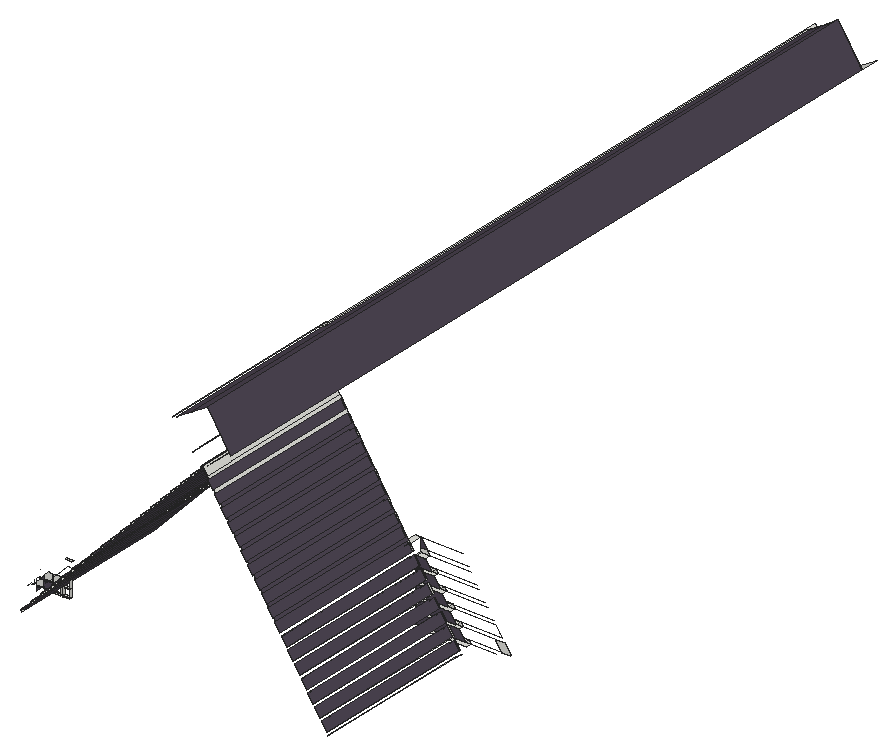
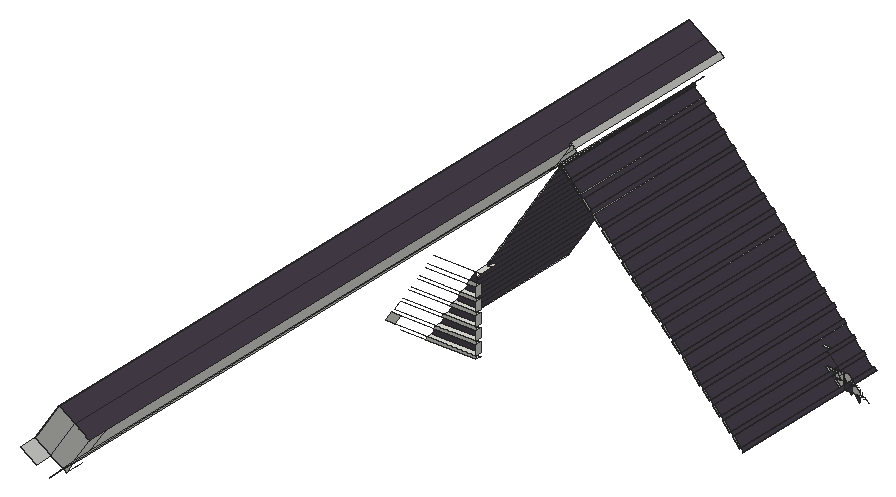
# SketchUp Ruby script. Lengths in inches.
U = 1.inch
M = Sketchup.active_model
def pt(a) = Geom::Point3d.new(a.map { |v| v * U })
def face(e, loops, mat)
  f = e.add_face(loops[0].map { |a| pt(a) })
  loops[1..].each { |l| e.add_face(l.map { |a| pt(a) }).erase! }
  f.material = f.back_material = mat if mat
  f
end
# faces: each face lists its corners as indices into pts; further lists are holes
def faces(e, pts, list, mat = nil) = list.each { |f| face(e, (f[0].is_a?(Array) ? f : [f]).map { |l| l.map { |i| pts[i] } }, mat) }
# xy, xz, yz: faces in a plane at the given z, y or x. An outline is a flat list of corners, or four numbers for a rectangle; further outlines are holes
def ring(l) = l.size == 4 ? [[l[0], l[1]], [l[2], l[1]], [l[2], l[3]], [l[0], l[3]]] : l.each_slice(2).to_a
def flat(e, list, mat, &to3) = list.each { |f| face(e, (f[0].is_a?(Array) ? f : [f]).map { |l| ring(l).map { |u, v| to3.(u, v) } }, mat) }
def xy(e, z, list, mat = nil) = flat(e, list, mat) { |x, y| [x, y, z] }
def xz(e, y, list, mat = nil) = flat(e, list, mat) { |x, z| [x, y, z] }
def yz(e, x, list, mat = nil) = flat(e, list, mat) { |y, z| [x, y, z] }
def lines(e, pts, list) = list.each { |a, b| e.add_line(pt(pts[a]), pt(pts[b])) }
# prism: a flat outline (further loops are holes) pulled along v
def prism(e, loops, v, mat = nil)
  f = face(e, loops, mat); d = Geom::Vector3d.new(v.map { |x| x * U })
  f.pushpull(f.normal.samedirection?(d) ? d.length : -d.length)
end
def box(e, o, s, mat = nil) = prism(e, [[o, [o[0] + s[0], o[1], o[2]], [o[0] + s[0], o[1] + s[1], o[2]], [o[0], o[1] + s[1], o[2]]]], [0, 0, s[2]], mat)
def at(x, y, z, deg = 0) = Geom::Transformation.translation(pt([x, y, z])) * Geom::Transformation.rotation(ORIGIN, Z_AXIS, deg.degrees)
def axes(o, x, y, z) = Geom::Transformation.new([*x, 0, *y, 0, *z, 0, *pt(o).to_a, 1])
def part(name) = M.definitions.add(name)
# library, detail: a bought-in or finely detailed component or shape, given as its bounding box
def library(name, o, s) = part(name).tap { |d| box(d.entities, o, s) }
def detail(e, o, s) = box(e.add_group.entities, o, s)
def put(e, d, t, mat = nil) = e.add_instance(d, t).tap { |i| i.material = mat if mat }
def group(e, t, mat = nil) = e.add_group.tap { |g| g.transformation = t; g.material = mat if mat }.entities
root = M.entities
M.materials.add("[Color M06]").color = [79, 71, 84]
xy(root,386.372,[[1096.787,2376.244,1113.36,2378.119]])
xy(root,386.399,[[1013.083,2332.135,1015.395,2332.76],[1015.995,2332.135,1018.307,2332.76]])
xy(root,386.837,[[1013.267,2332.135,1015.395,2332.76],[1015.995,2332.135,1018.307,2332.76]])
xy(root,387.495,[[1096.787,2376.244,1112.64,2378.119]])
xy(root,389.149,[[1015.995,2332.135,1018.307,2332.76]])
xy(root,389.587,[[1015.995,2332.135,1018.307,2332.76]])
xy(root,390.622,[[1096.787,2376.244,1110.635,2378.119]])
xy(root,391.745,[[1096.787,2376.244,1109.915,2378.119]])
xy(root,391.899,[[1018.012,2332.135,1018.307,2332.76]])
xy(root,394.872,[[1096.787,2376.244,1107.911,2378.119]])
xy(root,395.995,[[1096.787,2376.244,1107.191,2378.119]])
xy(root,397.749,[[1016.769,2332.135,1019.019,2332.76]])
xy(root,399.122,[[1096.787,2376.244,1105.186,2378.119]])
xy(root,400.245,[[1096.787,2376.244,1104.466,2378.119]])
xy(root,403.372,[[1096.787,2376.244,1102.461,2378.119]])
xy(root,404.495,[[1096.787,2376.244,1101.741,2378.119]])
xy(root,407.622,[[1096.787,2376.244,1099.736,2378.119]])
xy(root,412.223,[[1095.037,2371.682,1096.787,2373.557],[1095.037,2373.557,1096.787,2378.119]])
xz(root,2319.182,[[1073.488,447.754,1073.856,447.99,1072.287,450.4375,1071.978,450.109],[1071.978,450.109,1072.287,450.4375,1071.919,450.201]])
xz(root,2332.135,[[1007.259,385.926,1007.702,386.399,1007.259,386.399],[1010.171,386.283,1010.28,386.399,1010.171,386.399],[1006.497,386.837,1006.659,386.837,1006.659,387.008],[1007.259,386.837,1009.091,386.837,1009.571,387.346,1009.571,389.149,1008.674,389.149,1007.259,387.645],[1009.091,386.837,1009.571,386.837,1009.571,387.346],
  [1013.083,386.837,1013.267,386.837,1015.395,389.107,1015.395,389.149,1013.083,389.149],[1010.171,389.033,1010.28,389.149,1010.171,389.149],[1009.086,389.587,1009.571,389.587,1009.571,390.102],[1010.171,389.587,1011.68,389.587,1012.483,390.44,1012.483,391.899,1011.263,391.899,1010.171,390.739],[1011.68,389.587,1012.483,389.587,1012.483,390.44],
  [1013.083,389.587,1013.267,389.587,1015.395,391.857,1015.395,391.899,1013.857,391.899,1013.083,391.077],[1013.267,389.587,1015.395,389.587,1015.395,391.857],[1015.995,389.747,1018.012,391.899,1015.995,391.899],[1013.083,391.077,1013.857,391.899,1013.083,391.899]])
xz(root,2332.135,[[1007.259,384.89,1008.68,386.399,1007.702,386.399,1007.259,385.926],[1010.171,386.837,1012.483,386.837,1012.483,389.149,1011.268,389.149,1010.171,387.983,1009.571,387.346,1009.571,389.149,1008.674,389.149,1009.086,389.587,1009.571,389.587,1009.571,390.102,1010.171,390.739,1010.171,389.587,1011.68,389.587,1011.268,389.149,1010.171,389.149]],"[Color M06]")
xz(root,2371.682,[[1113.509,385.328,1113.453,385.417,1113.821,385.653,1113.878,385.565],[1111.317,388.748,1111.26,388.837,1111.628,389.073,1111.685,388.985],[1109.124,392.168,1109.068,392.257,1109.436,392.493,1109.493,392.405],[1106.932,395.588,1106.875,395.677,1107.243,395.913,1107.3,395.825],[1104.739,399.009,1104.682,399.097,1105.051,399.333,1105.107,399.245],
  [1102.547,402.429,1102.49,402.517,1102.858,402.753,1102.915,402.665],[1100.354,405.849,1100.297,405.937,1100.665,406.173,1100.722,406.085],[1098.161,409.269,1098.105,409.357,1098.473,409.593,1098.53,409.505],[1095.969,412.689,1095.912,412.777,1096.28,413.013,1096.337,412.925],[1093.776,416.109,1093.719,416.197,1094.088,416.433,1094.144,416.345],
  [1091.584,419.529,1091.527,419.617,1091.895,419.853,1091.952,419.765],[1089.391,422.949,1089.334,423.037,1089.702,423.273,1089.759,423.185],[1087.198,426.369,1087.142,426.457,1087.51,426.693,1087.567,426.605],[1085.006,429.789,1084.949,429.877,1085.317,430.113,1085.374,430.025],[1082.813,433.209,1082.756,433.297,1083.125,433.533,1083.181,433.445],
  [1080.621,436.629,1080.564,436.717,1080.932,436.953,1080.989,436.865],[1078.428,440.049,1078.371,440.137,1078.74,440.373,1078.796,440.285],[1076.235,443.469,1076.179,443.557,1076.547,443.793,1076.604,443.705],[1074.043,446.889,1073.986,446.977,1074.354,447.213,1074.411,447.125]])
xz(root,2373.557,[[1112.955,386.194,1111.317,388.748,1111.685,388.985,1113.323,386.43],[1013.667,387.25,1016.089,389.822,1015.633,390.251,1013.212,387.679],[1110.762,389.614,1109.124,392.168,1109.493,392.405,1111.13,389.85],[1016.966,390.754,1019.387,393.327,1018.932,393.755,1016.511,391.183],[1108.569,393.034,1106.932,395.588,1107.3,395.825,1108.938,393.27],
  [1020.265,394.259,1022.686,396.831,1022.231,397.259,1019.809,394.687],[1106.377,396.454,1104.739,399.009,1105.107,399.245,1106.745,396.69],[1023.563,397.763,1025.984,400.335,1025.529,400.763,1023.108,398.191],[1104.184,399.874,1102.547,402.429,1102.915,402.665,1104.553,400.11],[1026.862,401.267,1029.283,403.839,1028.828,404.268,1026.407,401.696],
  [1101.992,403.294,1100.354,405.849,1100.722,406.085,1102.36,403.53],[1030.16,404.771,1032.581,407.344,1032.126,407.772,1029.705,405.2],[1099.799,406.714,1098.161,409.269,1098.53,409.505,1100.167,406.95],[1033.459,408.276,1035.88,410.848,1035.425,411.276,1033.004,408.704],[1097.606,410.134,1096.419,411.987,1096.787,412.223,1097.975,410.37],
  [1036.757,411.78,1039.178,414.352,1038.723,414.78,1036.302,412.208],[1096.419,411.987,1096.267,412.223,1096.787,412.223],[1096.267,412.223,1096.787,412.223,1096.337,412.925,1095.969,412.689],[1095.414,413.554,1095.782,413.79,1094.594,415.643,1094.226,415.407],[1040.056,415.284,1042.477,417.856,1042.022,418.285,1039.601,415.713],
  [1094.226,415.407,1094.594,415.643,1094.144,416.345,1093.776,416.109],[1093.221,416.974,1093.59,417.21,1092.402,419.063,1092.033,418.827],[1043.354,418.788,1045.775,421.361,1045.32,421.789,1042.899,419.217],[1092.033,418.827,1092.402,419.063,1091.952,419.765,1091.584,419.529],[1091.029,420.394,1091.397,420.63,1090.209,422.483,1089.841,422.247],
  [1089.841,422.247,1090.209,422.483,1089.759,423.185,1089.391,422.949],[1046.653,422.293,1049.074,424.865,1048.619,425.293,1046.198,422.721],[1088.836,423.814,1089.204,424.05,1088.017,425.903,1087.648,425.667],[1087.648,425.667,1088.017,425.903,1087.567,426.605,1087.198,426.369],[1049.951,425.797,1052.373,428.369,1051.917,428.797,1049.496,426.225],
  [1086.643,427.234,1087.012,427.47,1085.824,429.323,1085.456,429.087],[1085.456,429.087,1085.824,429.323,1085.374,430.025,1085.006,429.789],[1053.25,429.301,1055.671,431.873,1055.216,432.302,1052.795,429.73],[1084.451,430.654,1084.819,430.89,1083.631,432.743,1083.263,432.507],[1083.263,432.507,1083.631,432.743,1083.181,433.445,1082.813,433.209],
  [1056.549,432.805,1058.97,435.378,1058.515,435.806,1056.093,433.234],[1082.258,434.074,1082.627,434.31,1081.439,436.163,1081.07,435.927],[1081.07,435.927,1081.439,436.163,1080.989,436.865,1080.621,436.629],[1059.847,436.31,1062.268,438.882,1061.813,439.31,1059.392,436.738],[1080.066,437.494,1080.434,437.73,1079.246,439.583,1078.878,439.347],
  [1078.878,439.347,1079.246,439.583,1078.796,440.285,1078.428,440.049],[1063.146,439.814,1065.567,442.386,1065.112,442.814,1062.69,440.242],[1077.873,440.914,1078.241,441.15,1077.054,443.003,1076.685,442.767],[1076.685,442.767,1077.054,443.003,1076.604,443.705,1076.235,443.469],[1066.444,443.318,1068.865,445.89,1068.41,446.319,1065.989,443.747],
  [1075.68,444.334,1076.049,444.57,1074.861,446.423,1074.493,446.187],[1074.493,446.187,1074.861,446.423,1074.411,447.125,1074.043,446.889],[1069.743,446.822,1072.164,449.395,1071.709,449.823,1069.288,447.251],[1073.488,447.754,1073.856,447.99,1072.668,449.843,1072.3,449.607],[1072.3,449.607,1072.668,449.843,1072.287,450.4375,1071.978,450.109],
  [1071.978,450.109,1071.919,450.201,1072.287,450.4375]])
xz(root,2376.244,[[1096.787,387.495,1112.64,387.495,1110.635,390.622,1096.787,390.622],[1096.787,391.745,1109.915,391.745,1107.911,394.872,1096.787,394.872],[1096.787,395.995,1107.191,395.995,1105.186,399.122,1096.787,399.122],[1096.787,400.245,1104.466,400.245,1102.461,403.372,1096.787,403.372],[1096.787,404.495,1101.741,404.495,1099.736,407.622,1096.787,407.622]],"[Color M06]")
xz(root,2378.119,[[1096.787,386.372,1113.36,386.372,1112.64,387.495,1096.787,387.495],[1123.539,387.495,1126.264,387.495,1124.259,390.622,1121.534,390.622],[1096.787,390.622,1110.635,390.622,1109.915,391.745,1096.787,391.745],[1096.787,394.872,1107.911,394.872,1107.191,395.995,1096.787,395.995],[1096.787,399.122,1105.186,399.122,1104.466,400.245,1096.787,400.245],
  [1096.787,403.372,1102.461,403.372,1101.741,404.495,1096.787,404.495],[1096.787,407.622,1099.736,407.622,1098.856,408.995,1096.787,408.995],[1096.787,412.122,1096.851,412.122,1096.787,412.223]])
xz(root,2378.119,[[1096.787,408.995,1098.856,408.995,1096.851,412.122,1096.787,412.122]],"[Color M06]")
xz(root,2380.477,[[1069.147,453.393,1061.61,460.488,1062.381,461.307,1066.649,457.29],[1069.147,453.393,1066.649,457.29,1069.918,454.213],[1069.918,454.213,1066.649,457.29,1067.977,458.7,1071.246,455.623],[1066.649,457.29,1062.381,461.307,1063.709,462.718,1067.977,458.7]])
xz(root,2571.585,[[1069.093,453.336,1069.147,453.393,1069.082,453.352]])
xz(root,2578.119,[[1071.34,449.83,1069.093,453.336,1069.147,453.393,1072.287,450.4375],[1072.287,450.4375,1069.147,453.393,1063.728,461.846,1068.662,465.009,1076.339,453.035],[1076.339,453.035,1068.662,465.009,1073.923,468.382,1081.6,456.408],[1069.093,453.336,1069.082,453.352,1069.147,453.393]])
yz(root,1015.395,[[2332.135,386.837,2332.76,389.107]])
yz(root,1015.995,[[2332.135,386.837,2332.76,389.149],[2332.135,389.587,2332.76,389.747]])
yz(root,1018.307,[[2332.135,386.837,2332.76,389.149],[2332.135,389.587,2332.76,391.899]])
yz(root,1096.787,[[2376.244,387.495,2378.119,390.622],[2376.244,391.745,2378.119,394.872],[2376.244,395.995,2378.119,399.122],[2376.244,400.245,2378.119,403.372],[2376.244,404.495,2378.119,407.622]])
p = [[1113.878,2371.682,385.565],[1113.878,2373.557,385.565],[1113.509,2373.557,385.328],[1113.509,2371.682,385.328],[1113.821,2319.182,385.653],[1113.821,2371.682,385.653],
  [1113.453,2371.682,385.417],[1113.453,2319.182,385.417],[1111.26,2319.182,388.837],[1111.26,2371.682,388.837],[1111.317,2371.682,388.748],[1111.317,2373.557,388.748],
  [1112.955,2373.557,386.194],[1112.955,2319.182,386.194],[1113.323,2373.557,386.43],[1113.323,2319.182,386.43],[1012.335,2373.557,386.746],[1012.335,2319.182,386.746],
  [1012.79,2319.182,386.318],[1012.79,2373.557,386.318],[1013.212,2373.557,387.679],[1013.212,2319.182,387.679],[1015.395,2332.135,389.107],[1013.267,2332.135,386.837],
  [1013.267,2332.76,386.837],[1015.395,2332.76,389.107],[1013.667,2373.557,387.25],[1013.667,2319.182,387.25],[1016.089,2373.557,389.822],[1016.089,2319.182,389.822],
  [1111.685,2371.682,388.985],[1111.685,2373.557,388.985],[1111.628,2319.182,389.073],[1111.628,2371.682,389.073],[1109.068,2319.182,392.257],[1109.068,2371.682,392.257],
  [1109.124,2371.682,392.168],[1109.124,2373.557,392.168],[1110.762,2373.557,389.614],[1110.762,2319.182,389.614],[1111.13,2373.557,389.85],[1111.13,2319.182,389.85],
  [1018.012,2332.135,391.899],[1015.995,2332.135,389.747],[1015.995,2332.76,389.747],[1018.012,2332.76,391.899],[1015.633,2373.557,390.251],[1015.633,2319.182,390.251],
  [1016.511,2373.557,391.183],[1016.511,2319.182,391.183],[1016.966,2373.557,390.754],[1016.966,2319.182,390.754],[1019.387,2373.557,393.327],[1019.387,2319.182,393.327],
  [1109.493,2371.682,392.405],[1109.493,2373.557,392.405],[1109.436,2319.182,392.493],[1109.436,2371.682,392.493],[1106.875,2319.182,395.677],[1106.875,2371.682,395.677],
  [1106.932,2371.682,395.588],[1106.932,2373.557,395.588],[1108.569,2373.557,393.034],[1108.569,2319.182,393.034],[1108.938,2373.557,393.27],[1108.938,2319.182,393.27],
  [1018.932,2373.557,393.755],[1018.932,2319.182,393.755],[1019.809,2373.557,394.687],[1019.809,2319.182,394.687],[1020.265,2373.557,394.259],[1020.265,2319.182,394.259],
  [1022.686,2373.557,396.831],[1022.686,2319.182,396.831],[1107.3,2371.682,395.825],[1107.3,2373.557,395.825],[1107.243,2319.182,395.913],[1107.243,2371.682,395.913],
  [1104.682,2319.182,399.097],[1104.682,2371.682,399.097],[1104.739,2371.682,399.009],[1104.739,2373.557,399.009],[1106.377,2373.557,396.454],[1106.377,2319.182,396.454],
  [1106.745,2373.557,396.69],[1106.745,2319.182,396.69],[1022.231,2373.557,397.259],[1022.231,2319.182,397.259],[1023.108,2373.557,398.191],[1023.108,2319.182,398.191],
  [1023.563,2373.557,397.763],[1023.563,2319.182,397.763],[1025.984,2373.557,400.335],[1025.984,2319.182,400.335],[1105.107,2371.682,399.245],[1105.107,2373.557,399.245],
  [1105.051,2319.182,399.333],[1105.051,2371.682,399.333],[1102.49,2319.182,402.517],[1102.49,2371.682,402.517],[1102.547,2371.682,402.429],[1102.547,2373.557,402.429],
  [1104.184,2373.557,399.874],[1104.184,2319.182,399.874],[1104.553,2373.557,400.11],[1104.553,2319.182,400.11],[1025.529,2373.557,400.763],[1025.529,2319.182,400.763],
  [1026.407,2373.557,401.696],[1026.407,2319.182,401.696],[1026.862,2373.557,401.267],[1026.862,2319.182,401.267],[1029.283,2373.557,403.839],[1029.283,2319.182,403.839],
  [1102.915,2371.682,402.665],[1102.915,2373.557,402.665],[1102.858,2319.182,402.753],[1102.858,2371.682,402.753],[1100.297,2319.182,405.937],[1100.297,2371.682,405.937],
  [1100.354,2371.682,405.849],[1100.354,2373.557,405.849],[1101.992,2373.557,403.294],[1101.992,2319.182,403.294],[1102.36,2373.557,403.53],[1102.36,2319.182,403.53],
  [1028.828,2373.557,404.268],[1028.828,2319.182,404.268],[1029.705,2373.557,405.2],[1029.705,2319.182,405.2],[1030.16,2373.557,404.771],[1030.16,2319.182,404.771],
  [1032.581,2373.557,407.344],[1032.581,2319.182,407.344],[1100.722,2371.682,406.085],[1100.722,2373.557,406.085],[1100.665,2319.182,406.173],[1100.665,2371.682,406.173],
  [1098.105,2319.182,409.357],[1098.105,2371.682,409.357],[1098.161,2371.682,409.269],[1098.161,2373.557,409.269],[1099.799,2373.557,406.714],[1099.799,2319.182,406.714],
  [1100.167,2373.557,406.95],[1100.167,2319.182,406.95],[1032.126,2373.557,407.772],[1032.126,2319.182,407.772],[1033.004,2373.557,408.704],[1033.004,2319.182,408.704],
  [1033.459,2373.557,408.276],[1033.459,2319.182,408.276],[1035.88,2373.557,410.848],[1035.88,2319.182,410.848],[1098.53,2371.682,409.505],[1098.53,2373.557,409.505],
  [1098.473,2319.182,409.593],[1098.473,2371.682,409.593],[1095.912,2319.182,412.777],[1095.912,2371.682,412.777],[1095.969,2371.682,412.689],[1095.969,2373.557,412.689],
  [1096.267,2373.557,412.223],[1096.419,2373.557,411.987],[1097.606,2373.557,410.134],[1097.606,2319.182,410.134],[1097.975,2373.557,410.37],[1097.975,2319.182,410.37],
  [1035.425,2373.557,411.276],[1035.425,2319.182,411.276],[1036.302,2373.557,412.208],[1036.302,2319.182,412.208],[1036.757,2373.557,411.78],[1036.757,2319.182,411.78],
  [1039.178,2373.557,414.352],[1039.178,2319.182,414.352],[1096.337,2371.682,412.925],[1096.337,2373.557,412.925],[1096.28,2319.182,413.013],[1096.28,2371.682,413.013],
  [1095.782,2319.182,413.79],[1095.782,2373.557,413.79],[1093.719,2319.182,416.197],[1093.719,2371.682,416.197],[1093.776,2371.682,416.109],[1093.776,2373.557,416.109],
  [1094.226,2373.557,415.407],[1095.414,2373.557,413.554],[1095.414,2319.182,413.554],[1038.723,2373.557,414.78],[1038.723,2319.182,414.78],[1039.601,2373.557,415.713],
  [1039.601,2319.182,415.713],[1040.056,2373.557,415.284],[1040.056,2319.182,415.284],[1042.477,2373.557,417.856],[1042.477,2319.182,417.856],[1094.144,2371.682,416.345],
  [1094.144,2373.557,416.345],[1094.088,2319.182,416.433],[1094.088,2371.682,416.433],[1093.59,2319.182,417.21],[1093.59,2373.557,417.21],[1091.527,2319.182,419.617],
  [1091.527,2371.682,419.617],[1091.584,2371.682,419.529],[1091.584,2373.557,419.529],[1092.033,2373.557,418.827],[1093.221,2373.557,416.974],[1093.221,2319.182,416.974],
  [1042.022,2373.557,418.285],[1042.022,2319.182,418.285],[1042.899,2373.557,419.217],[1042.899,2319.182,419.217],[1043.354,2373.557,418.788],[1043.354,2319.182,418.788],
  [1045.775,2373.557,421.361],[1045.775,2319.182,421.361],[1091.952,2371.682,419.765],[1091.952,2373.557,419.765],[1091.895,2319.182,419.853],[1091.895,2371.682,419.853],
  [1091.397,2319.182,420.63],[1091.397,2373.557,420.63],[1089.334,2319.182,423.037],[1089.334,2371.682,423.037],[1089.391,2371.682,422.949],[1089.391,2373.557,422.949],
  [1089.841,2373.557,422.247],[1091.029,2373.557,420.394],[1091.029,2319.182,420.394],[1045.32,2373.557,421.789],[1045.32,2319.182,421.789],[1046.198,2373.557,422.721],
  [1046.198,2319.182,422.721],[1046.653,2373.557,422.293],[1046.653,2319.182,422.293],[1049.074,2373.557,424.865],[1049.074,2319.182,424.865],[1089.759,2371.682,423.185],
  [1089.759,2373.557,423.185],[1089.702,2319.182,423.273],[1089.702,2371.682,423.273],[1089.204,2319.182,424.05],[1089.204,2373.557,424.05],[1087.142,2319.182,426.457],
  [1087.142,2371.682,426.457],[1087.198,2371.682,426.369],[1087.198,2373.557,426.369],[1087.648,2373.557,425.667],[1088.836,2373.557,423.814],[1088.836,2319.182,423.814],
  [1048.619,2373.557,425.293],[1048.619,2319.182,425.293],[1049.496,2373.557,426.225],[1049.496,2319.182,426.225],[1049.951,2373.557,425.797],[1049.951,2319.182,425.797],
  [1052.373,2373.557,428.369],[1052.373,2319.182,428.369],[1087.567,2371.682,426.605],[1087.567,2373.557,426.605],[1087.51,2319.182,426.693],[1087.51,2371.682,426.693],
  [1087.012,2319.182,427.47],[1087.012,2373.557,427.47],[1084.949,2319.182,429.877],[1084.949,2371.682,429.877],[1085.006,2371.682,429.789],[1085.006,2373.557,429.789],
  [1085.456,2373.557,429.087],[1086.643,2373.557,427.234],[1086.643,2319.182,427.234],[1051.917,2373.557,428.797],[1051.917,2319.182,428.797],[1052.795,2373.557,429.73],
  [1052.795,2319.182,429.73],[1053.25,2373.557,429.301],[1053.25,2319.182,429.301],[1055.671,2373.557,431.873],[1055.671,2319.182,431.873],[1085.374,2371.682,430.025],
  [1085.374,2373.557,430.025],[1085.317,2319.182,430.113],[1085.317,2371.682,430.113],[1084.819,2319.182,430.89],[1084.819,2373.557,430.89],[1082.756,2319.182,433.297],
  [1082.756,2371.682,433.297],[1082.813,2371.682,433.209],[1082.813,2373.557,433.209],[1083.263,2373.557,432.507],[1084.451,2373.557,430.654],[1084.451,2319.182,430.654],
  [1055.216,2373.557,432.302],[1055.216,2319.182,432.302],[1056.093,2373.557,433.234],[1056.093,2319.182,433.234],[1056.549,2373.557,432.805],[1056.549,2319.182,432.805],
  [1058.97,2373.557,435.378],[1058.97,2319.182,435.378],[1083.181,2371.682,433.445],[1083.181,2373.557,433.445],[1083.125,2319.182,433.533],[1083.125,2371.682,433.533],
  [1082.627,2319.182,434.31],[1082.627,2373.557,434.31],[1080.564,2319.182,436.717],[1080.564,2371.682,436.717],[1080.621,2371.682,436.629],[1080.621,2373.557,436.629],
  [1081.07,2373.557,435.927],[1082.258,2373.557,434.074],[1082.258,2319.182,434.074],[1058.515,2373.557,435.806],[1058.515,2319.182,435.806],[1059.392,2373.557,436.738],
  [1059.392,2319.182,436.738],[1059.847,2373.557,436.31],[1059.847,2319.182,436.31],[1062.268,2373.557,438.882],[1062.268,2319.182,438.882],[1080.989,2371.682,436.865],
  [1080.989,2373.557,436.865],[1080.932,2319.182,436.953],[1080.932,2371.682,436.953],[1080.434,2319.182,437.73],[1080.434,2373.557,437.73],[1078.371,2319.182,440.137],
  [1078.371,2371.682,440.137],[1078.428,2371.682,440.049],[1078.428,2373.557,440.049],[1078.878,2373.557,439.347],[1080.066,2373.557,437.494],[1080.066,2319.182,437.494],
  [1061.813,2373.557,439.31],[1061.813,2319.182,439.31],[1062.69,2373.557,440.242],[1062.69,2319.182,440.242],[1063.146,2373.557,439.814],[1063.146,2319.182,439.814],
  [1065.567,2373.557,442.386],[1065.567,2319.182,442.386],[1078.796,2371.682,440.285],[1078.796,2373.557,440.285],[1078.74,2319.182,440.373],[1078.74,2371.682,440.373],
  [1078.241,2319.182,441.15],[1078.241,2373.557,441.15],[1076.179,2319.182,443.557],[1076.179,2371.682,443.557],[1076.235,2371.682,443.469],[1076.235,2373.557,443.469],
  [1076.685,2373.557,442.767],[1077.873,2373.557,440.914],[1077.873,2319.182,440.914],[1065.112,2373.557,442.814],[1065.112,2319.182,442.814],[1065.989,2373.557,443.747],
  [1065.989,2319.182,443.747],[1066.444,2373.557,443.318],[1066.444,2319.182,443.318],[1068.865,2373.557,445.89],[1068.865,2319.182,445.89],[1076.604,2371.682,443.705],
  [1076.604,2373.557,443.705],[1076.547,2319.182,443.793],[1076.547,2371.682,443.793],[1076.049,2319.182,444.57],[1076.049,2373.557,444.57],[1073.986,2319.182,446.977],
  [1073.986,2371.682,446.977],[1074.043,2371.682,446.889],[1074.043,2373.557,446.889],[1074.493,2373.557,446.187],[1075.68,2373.557,444.334],[1075.68,2319.182,444.334],
  [1068.41,2373.557,446.319],[1068.41,2319.182,446.319],[1069.288,2373.557,447.251],[1069.288,2319.182,447.251],[1069.743,2373.557,446.822],[1069.743,2319.182,446.822],
  [1072.164,2373.557,449.395],[1072.164,2319.182,449.395],[1074.411,2371.682,447.125],[1074.411,2373.557,447.125],[1074.354,2319.182,447.213],[1074.354,2371.682,447.213],
  [1073.856,2319.182,447.99],[1073.856,2373.557,447.99],[1072.3,2373.557,449.607],[1073.488,2373.557,447.754],[1073.488,2319.182,447.754],[1071.978,2319.182,450.109],
  [1071.919,2319.182,450.201],[1071.919,2373.557,450.201],[1071.978,2373.557,450.109],[1072.668,2373.557,449.843],[1072.287,2373.557,450.4375],[1072.287,2319.182,450.4375],
  [1071.709,2373.557,449.823],[1071.709,2319.182,449.823],[1072.218,2373.557,450.545],[1072.162,2319.182,450.633],[1072.162,2371.682,450.633],[1072.218,2371.682,450.545],
  [1072.287,2380.477,450.4375],[1072.287,2571.585,450.4375],[1072.287,2578.119,450.4375],[1072.287,2583.74,450.4375],[1069.147,2583.74,453.393],[1069.147,2578.119,453.393],
  [1069.147,2571.585,453.393],[1069.147,2380.477,453.393],[1076.339,2578.119,453.035],[1081.6,2578.119,456.408],[1081.6,2584.196,456.408],[1076.339,2584.196,453.035],
  [1069.093,2571.585,453.336],[1069.093,2319.182,453.336],[1069.147,2319.182,453.393],[1061.61,2380.477,460.488],[1061.61,2583.74,460.488],[1066.649,2380.477,457.29],
  [1063.728,2380.477,461.846],[1063.728,2571.585,461.846],[1063.728,2578.119,461.846],[1069.082,2571.585,453.352],[1069.082,2578.119,453.352],[1081.6,2319.182,456.408],
  [1073.923,2578.119,468.382],[1073.923,2319.182,468.382],[1062.381,2380.477,461.307],[1062.381,2319.182,461.307],[1063.709,2319.182,462.718],[1063.709,2380.477,462.718],
  [1068.662,2578.119,465.009],[1063.728,2319.182,461.846],[1064.268,2319.182,462.192],[1068.662,2319.182,465.009],[1018.443,2332.135,395.86],[1017.585,2332.135,395.86],
  [1013.857,2332.135,391.899],[1071.246,2380.477,455.623],[1071.246,2319.182,455.623],[1009.086,2332.135,389.587],[1008.112,2332.135,389.587],[1076.339,2319.182,453.035],
  [1071.34,2571.585,449.83],[1071.34,2578.119,449.83],[1118.089,2378.119,395.995],[1115.365,2378.119,395.995],[1112.64,2378.119,395.995],[1109.915,2378.119,395.995],
  [1116.085,2378.119,399.122],[1118.809,2378.119,399.122],[1107.911,2378.119,394.872],[1110.635,2378.119,394.872],[1113.36,2378.119,403.372],[1116.085,2378.119,403.372],
  [1109.915,2378.119,408.995],[1107.191,2378.119,408.995],[1107.191,2378.119,395.995],[1102.461,2378.119,412.122],[1105.186,2378.119,412.122],[1115.365,2378.119,387.495],
  [1112.64,2378.119,387.495],[1109.915,2378.119,400.245],[1107.191,2378.119,400.245],[1099.736,2378.119,412.122],[1101.741,2378.119,408.995],[1098.856,2378.119,408.995],
  [1113.36,2378.119,399.122],[1096.851,2378.119,412.122],[1104.466,2378.119,400.245],[1105.186,2378.119,403.372],[1107.911,2378.119,403.372],[1107.911,2378.119,412.122],
  [1110.635,2378.119,412.122],[1118.089,2378.119,387.495],[1107.911,2378.119,399.122],[1110.635,2378.119,399.122],[1118.089,2378.119,400.245],[1115.365,2378.119,400.245],
  [1110.635,2378.119,403.372],[1120.814,2378.119,387.495],[1104.466,2378.119,408.995],[1123.539,2378.119,387.495],[1112.64,2378.119,408.995],[1118.809,2378.119,390.622],
  [1121.534,2378.119,390.622],[1105.186,2378.119,407.622],[1107.911,2378.119,407.622],[1110.635,2378.119,390.622],[1113.36,2378.119,390.622],[1113.36,2378.119,386.372],
  [1116.085,2378.119,386.372],[1110.635,2378.119,407.622],[1113.36,2378.119,407.622],[1104.466,2378.119,404.495],[1101.741,2378.119,404.495],[1118.809,2378.119,386.372],
  [1121.534,2378.119,386.372],[1102.461,2378.119,407.622],[1109.915,2378.119,404.495],[1107.191,2378.119,404.495],[1115.365,2378.119,404.495],[1112.64,2378.119,404.495],
  [1120.814,2378.119,395.995],[1006.497,2332.135,386.837],[1005.535,2332.135,386.837],[1007.702,2332.135,389.149],[1008.674,2332.135,389.149],[1007.259,2332.135,387.645],
  [1007.259,2332.135,388.676],[1006.659,2332.135,388.036],[1006.659,2332.135,387.008],[1008.674,2332.135,391.899],[1008.68,2332.135,391.899],[1005.125,2332.135,386.399],
  [1006.086,2332.135,386.399],[1004.347,2332.135,385.569],[1112.64,2378.119,400.245],[1105.186,2378.119,399.122],[1123.539,2378.119,391.745],[1120.814,2378.119,391.745],
  [1116.085,2378.119,390.622],[1113.36,2378.119,394.872],[1116.085,2378.119,394.872],[1118.089,2378.119,391.745],[1112.64,2378.119,391.745],[1109.915,2378.119,391.745],
  [1115.365,2378.119,391.745],[1118.809,2378.119,394.872],[1121.534,2378.119,394.872],[1099.736,2378.119,407.622],[1102.461,2378.119,403.372]]
faces(root,p,[[0,1,2,3],[4,5,6,7],[14,15,13,12],[16,17,18,19],[22,23,24,25],[30,31,11,10],[32,33,9,8],[40,41,39,38],
  [42,43,44,45],[46,47,29,28],[49,48,50,51],[54,55,37,36],[56,57,35,34],[64,65,63,62],[66,67,53,52],[69,68,70,71],
  [74,75,61,60],[76,77,59,58],[84,85,83,82],[86,87,73,72],[89,88,90,91],[94,95,81,80],[96,97,79,78],[104,105,103,102],
  [106,107,93,92],[114,115,101,100],[116,117,99,98],[124,125,123,122],[126,127,113,112],[134,135,121,120],[136,137,119,118],[144,145,143,142],
  [146,147,133,132],[154,155,141,140],[156,157,139,138],[166,167,165,164],[168,169,153,152],[176,177,161,160],[178,179,159,158],[181,180,188,187],
  [189,190,175,174],[197,198,185,184],[199,200,183,182],[202,201,209,208],[210,211,196,195],[218,219,206,205],[220,221,204,203],[223,222,230,229],
  [231,232,217,216],[239,240,227,226],[241,242,225,224],[244,243,251,250],[252,253,238,237],[260,261,248,247],[262,263,246,245],[265,264,272,271],
  [273,274,259,258],[276,275,277,278],[281,282,269,268],[283,284,267,266],[286,285,293,292],[294,295,280,279],[297,296,298,299],[302,303,290,289],
  [304,305,288,287],[307,306,314,313],[315,316,301,300],[318,317,319,320],[323,324,311,310],[325,326,309,308],[328,327,335,334],[336,337,322,321],
  [339,338,340,341],[344,345,332,331],[346,347,330,329],[357,358,343,342],[360,359,361,362],[365,366,353,352],[367,368,351,350],[367,369,370,366,365,368],
  [378,379,364,363],[381,380,382,383],[386,387,374,373],[388,389,372,371],[388,390,391,387,386,389],[391,399,400,401,390],[402,403,385,384],[395,403,402,398,400,401],
  [401,400,397,396],[404,400,401,405,406,407],[408,409,410,411,412,413,414,415],[416,417,418,419],[414,420,421,422,415],[423,415,414,413,412,424],[414,415,425,426,427],[413,414,427,428],
  [429,414,413,430],[434,435,436,437]])
faces(root,p,[[8,9,10,11,12,13],[16,20,21,17],[21,20,26,27],[26,28,29,27],[34,35,36,37,38,39],[46,48,49,47],[50,52,53,51],[58,59,60,61,62,63],
  [66,68,69,67],[70,72,73,71],[78,79,80,81,82,83],[86,88,89,87],[90,92,93,91],[98,99,100,101,102,103],[106,108,109,107],[109,108,110,111],
  [110,112,113,111],[118,119,120,121,122,123],[126,128,129,127],[129,128,130,131],[130,132,133,131],[138,139,140,141,142,143],[146,148,149,147],[149,148,150,151],
  [150,152,153,151],[158,159,160,161,162,163,164,165],[168,170,171,169],[171,170,172,173],[172,174,175,173],[178,180,181,177,176,179],[182,183,184,185,186,187,188],[189,191,192,190],
  [192,191,193,194],[193,195,196,194],[199,201,202,198,197,200],[203,204,205,206,207,208,209],[210,212,213,211],[213,212,214,215],[214,216,217,215],[220,222,223,219,218,221],
  [224,225,226,227,228,229,230],[231,233,234,232],[234,233,235,236],[235,237,238,236],[241,243,244,240,239,242],[245,246,247,248,249,250,251],[252,254,255,253],[255,254,256,257],
  [256,258,259,257],[262,264,265,261,260,263],[266,267,268,269,270,271,272],[273,275,276,274],[277,279,280,278],[283,285,286,282,281,284],[287,288,289,290,291,292,293],[294,296,297,295],
  [298,300,301,299],[304,306,307,303,302,305],[308,309,310,311,312,313,314],[315,317,318,316],[319,321,322,320],[325,327,328,324,323,326],[329,330,331,332,333,334,335],[336,338,339,337],
  [340,342,343,341],[346,348,349,345,344,347],[350,351,352,353,354,355,356],[349,348,356,355],[357,359,360,358],[361,363,364,362],[371,372,373,374,375,376,377],[370,369,377,376],
  [378,380,381,379],[382,384,385,383],[392,393,394,395,396,397,398],[391,390,394,393],[431,417,432,433],[438,428,427,426,439,440,441],[438,441,433,432]],"[Color M06]")
lines(root,p,[[442,443],[443,444],[445,446],[447,448],[449,416],[450,451],[452,453],[454,455],[456,457],[458,459],[460,461],[462,463],
  [453,454],[455,464],[465,466],[467,468],[469,470],[471,465],[472,473],[474,456],[475,471],[470,476],[477,478],[466,479],
  [479,480],[481,467],[482,483],[484,485],[486,460],[487,481],[463,488],[478,486],[488,472],[489,487],[490,462],[491,492],
  [493,494],[495,496],[497,498],[494,499],[499,500],[501,502],[498,503],[503,504],[505,493],[506,507],[508,509],[509,506],
  [507,501],[483,474],[510,452],[511,512],[513,514],[515,516],[517,518],[519,520],[521,522],[521,523],[524,469],[525,482],
  [526,527],[485,524],[528,491],[529,530],[496,528],[459,529],[527,531],[532,533],[531,534],[535,536],[530,535],[536,526],
  [537,505],[538,477],[534,532]])
